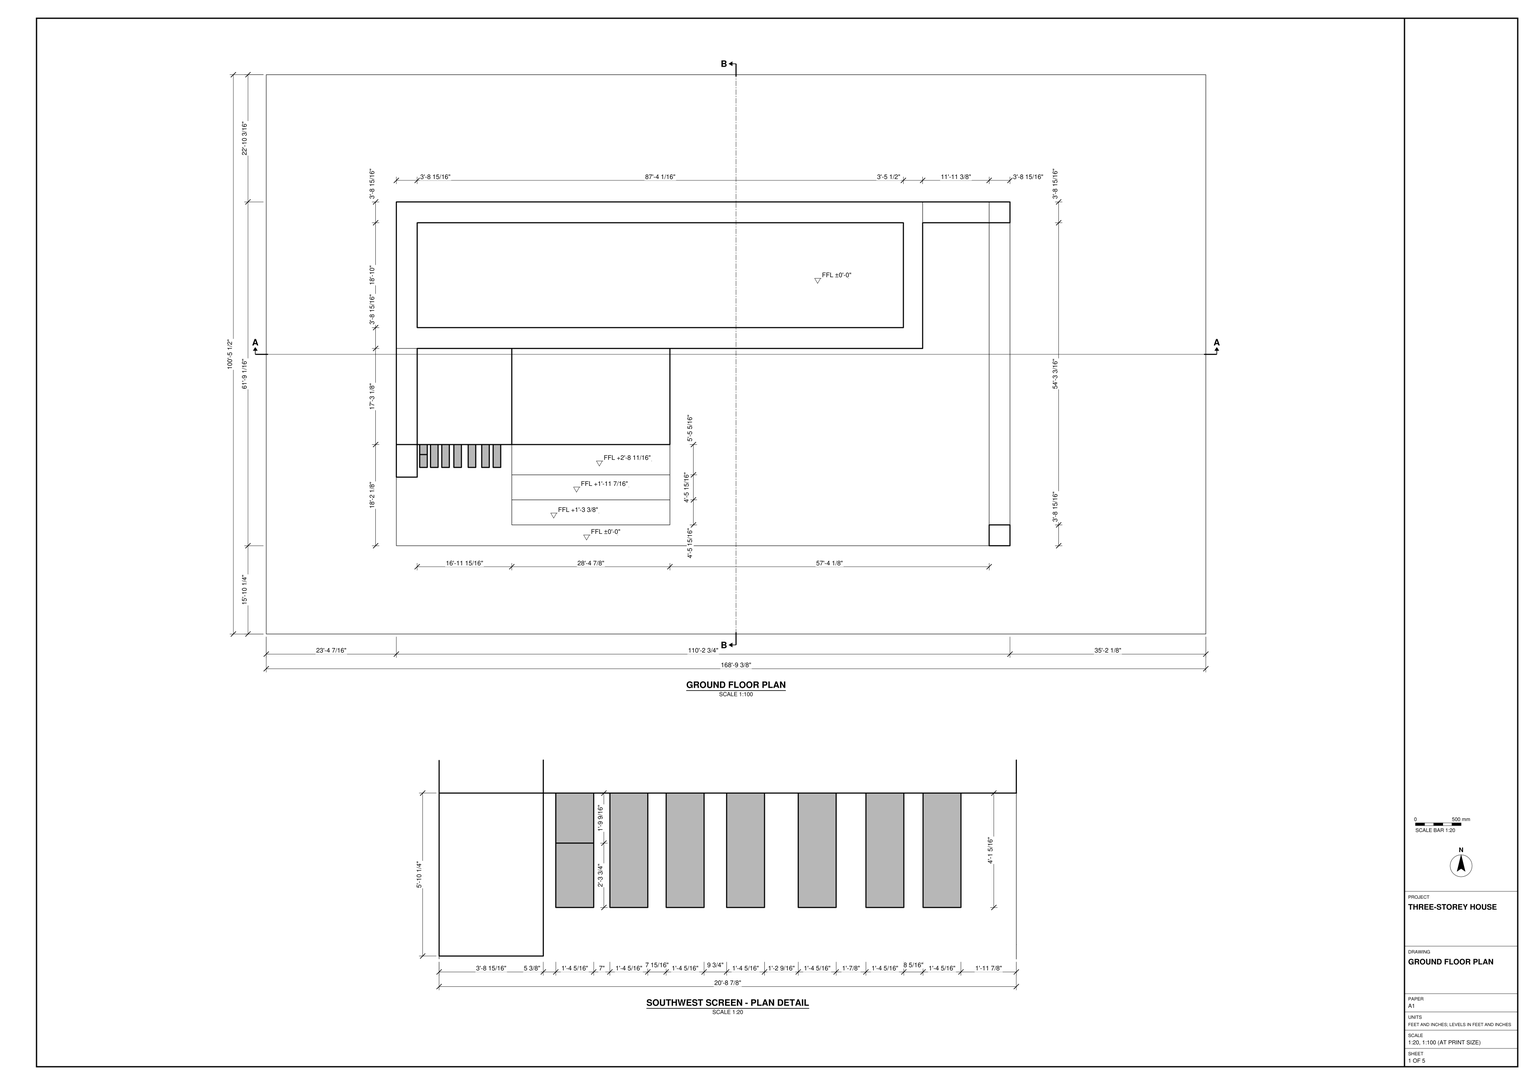
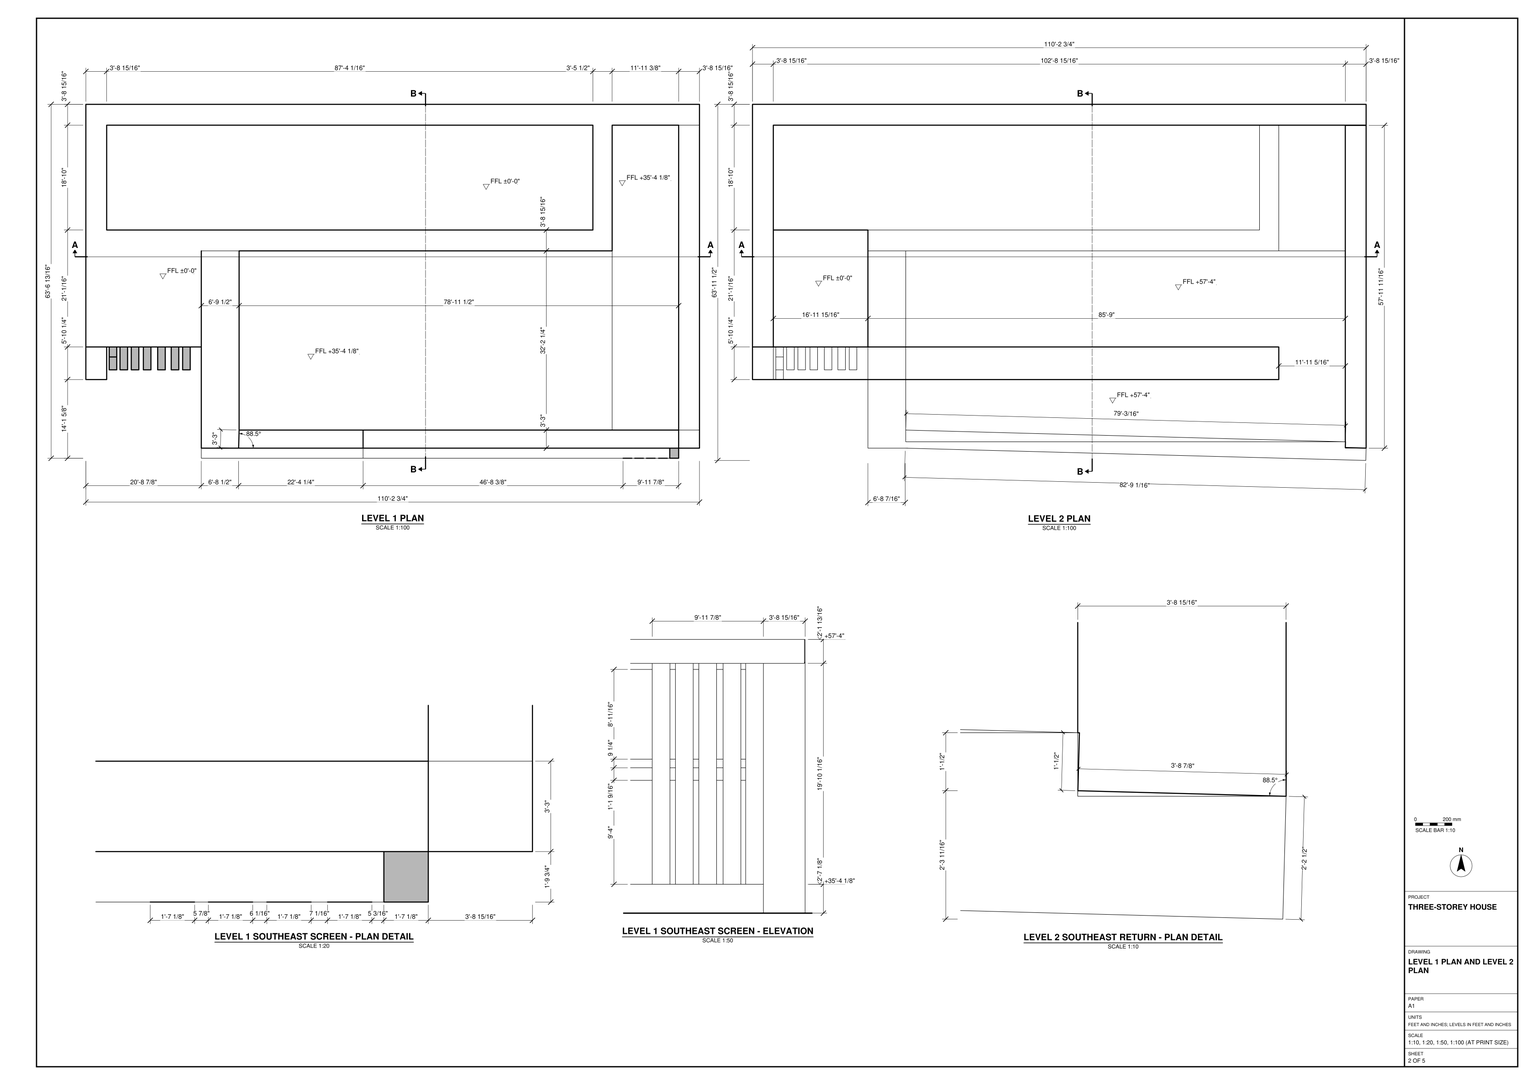
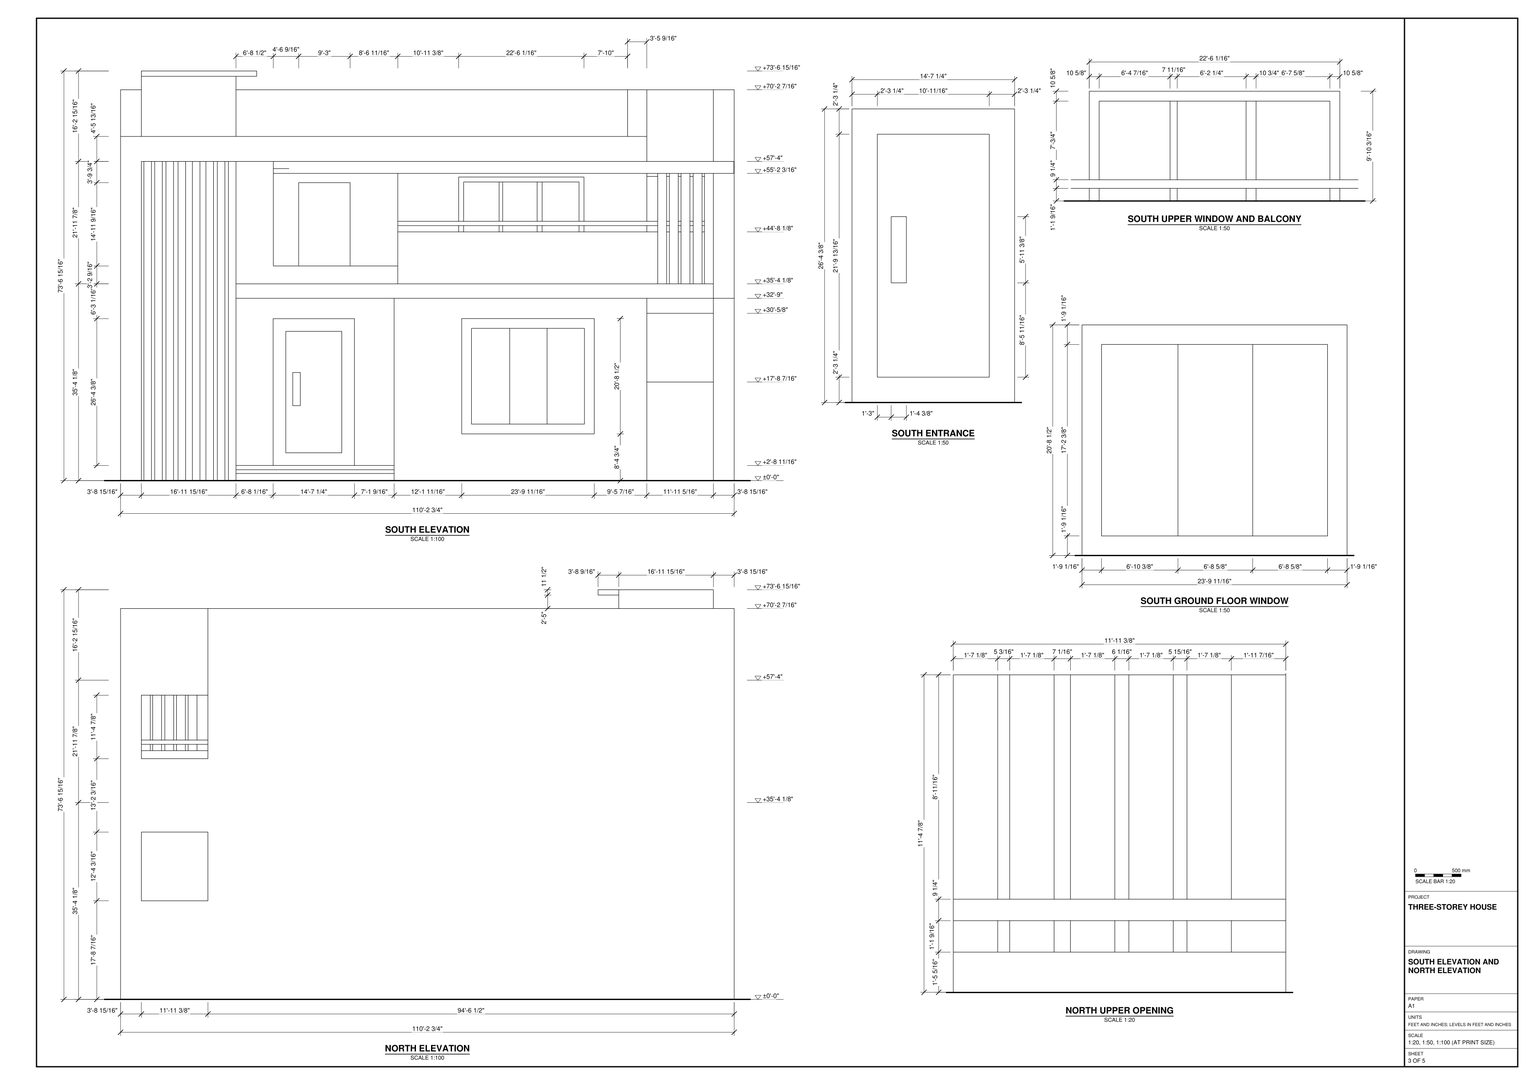
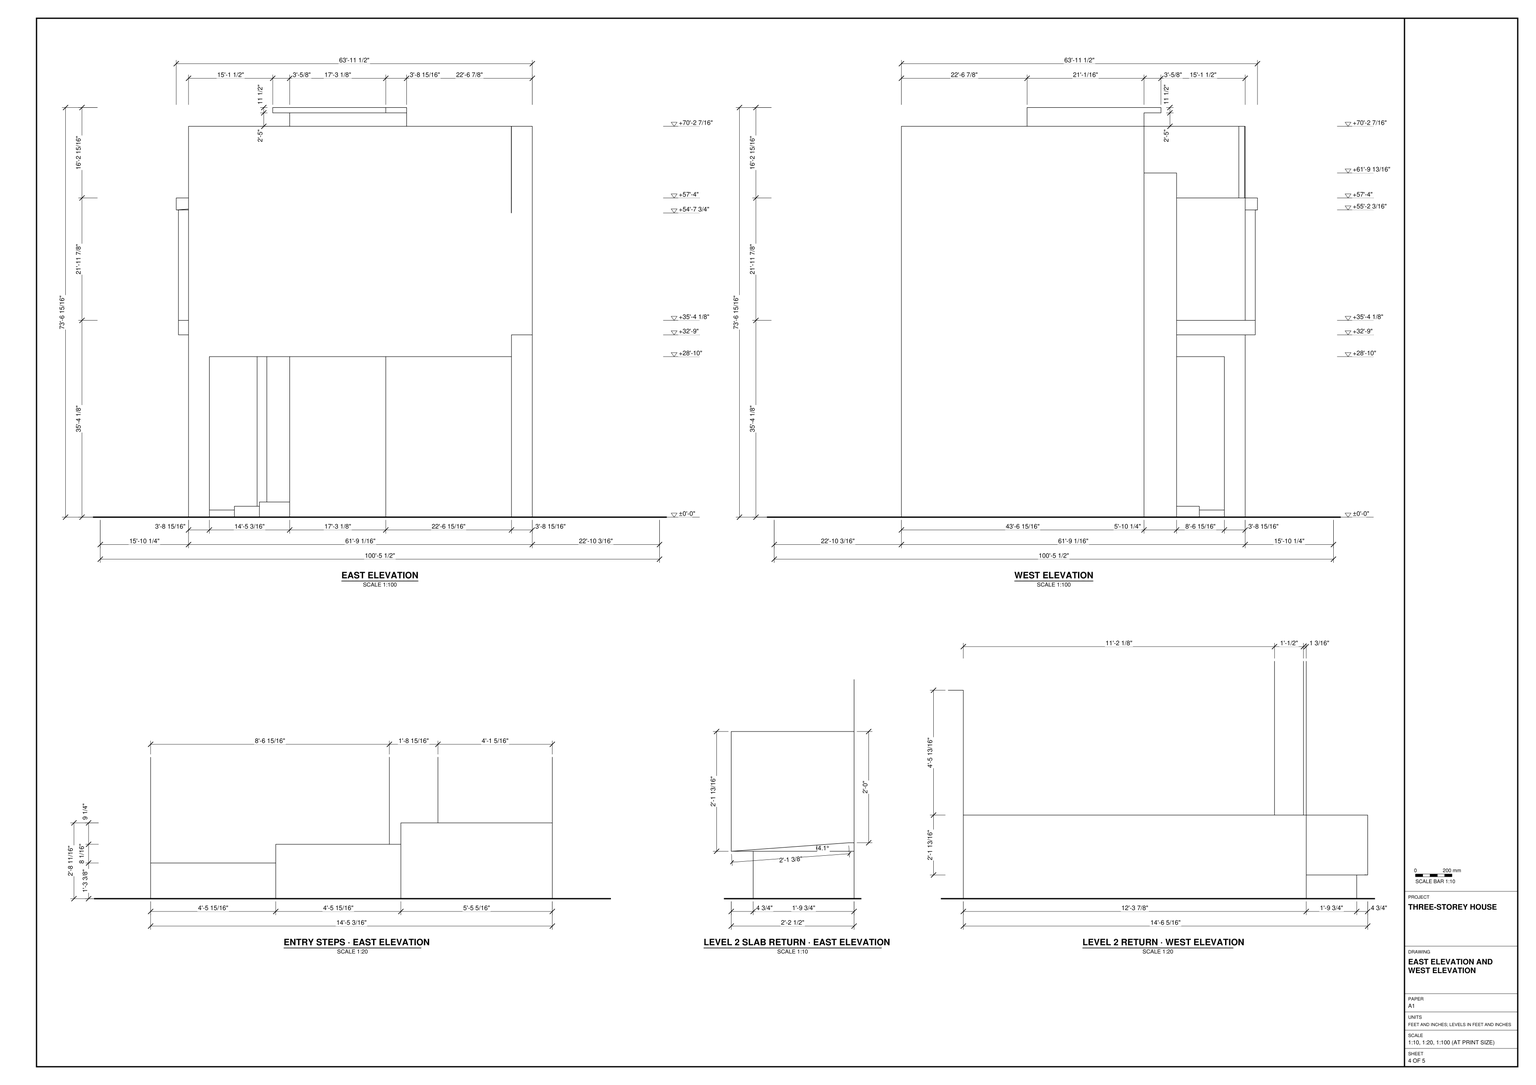
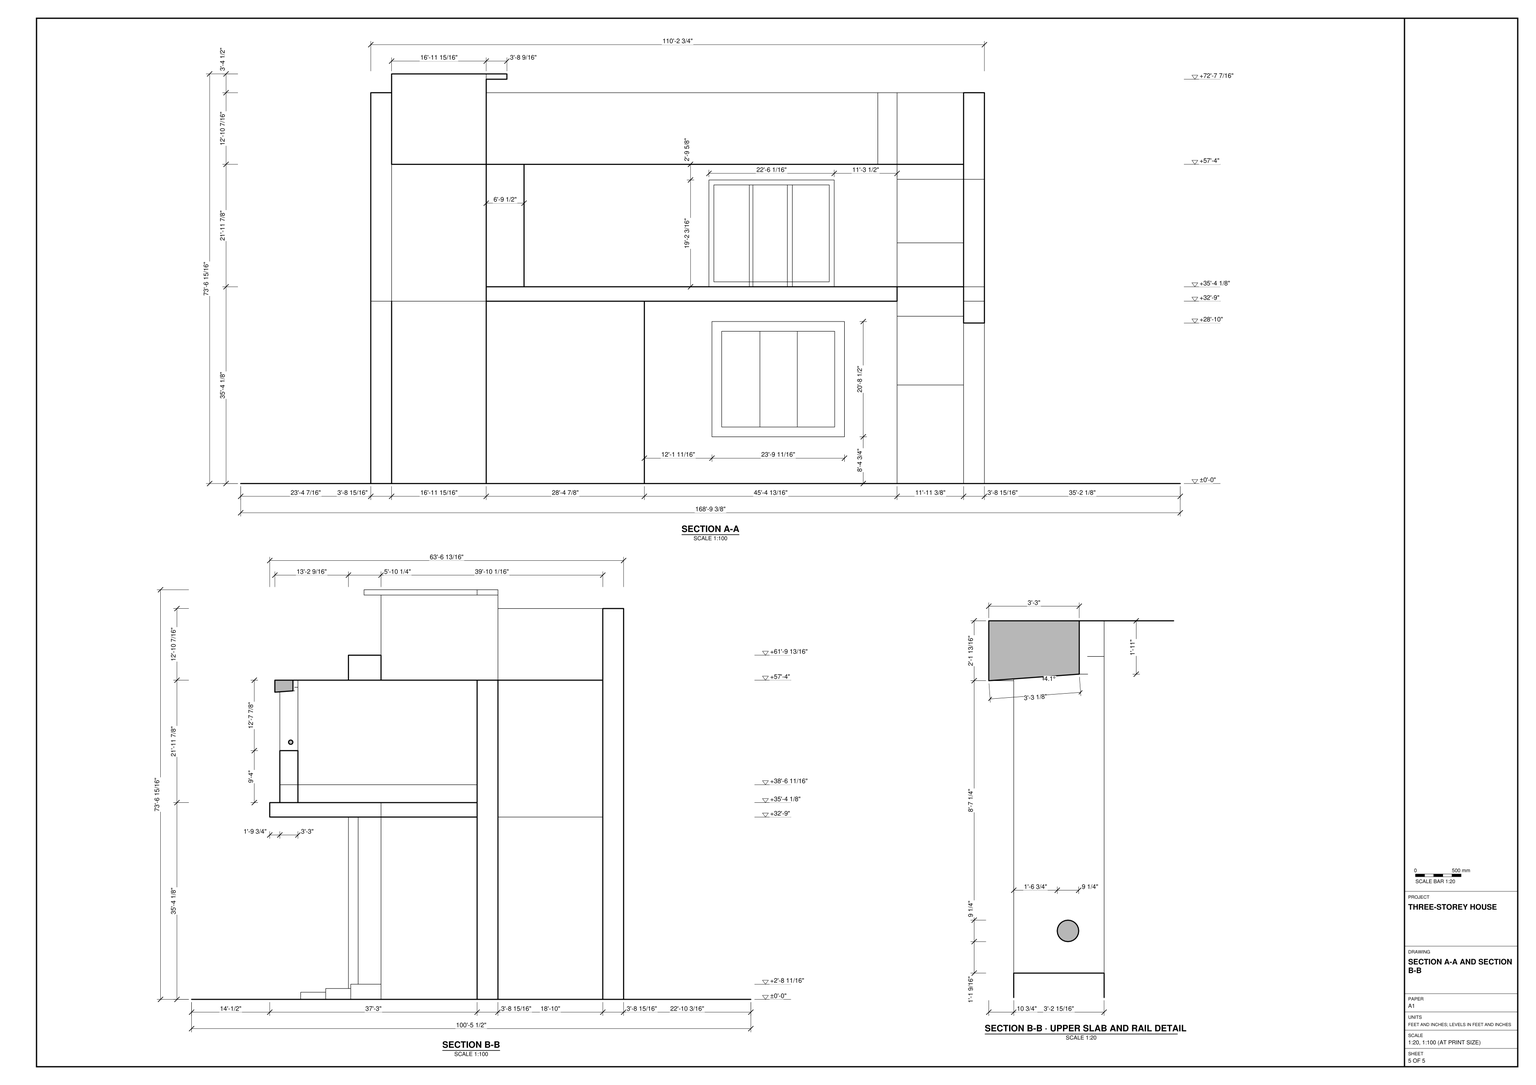
Build the three-storey house and its rectangular site base in SketchUp from task_files/diagram_01.pdf. Work in feet and inches. The overall model extents, including the base, are 168'-9 3/8" along X, 100'-5 1/2" along Y and 73'-6 15/16" along Z. Set the ground floor at ±0'-0", Level 1 at +35'-4 1/8" and Level 2 at +57'-4".

Position the house using the setbacks on the ground floor plan. Model the long rectangular space on the north side and follow the separate slab outlines and wall returns on the upper plans. Give the walls, floor slabs and roof their drawn thicknesses. Include the raised roof element and its projecting cap.

On the south side, run the broad entrance steps up to the framed door. Place the tall, spaced screen fins to the west of the steps and the divided ground floor window to the east of the door. Use the elevation details for the upper window, balcony edge and shorter southeast screen. On the north wall, align the lower opening with the screened opening above it. Include built-in joinery and main furniture only where shown. Decor and loose items may be any suitable library components.

Keep walls, slabs and roof elements in separate groups or components, group each furniture or joinery piece separately, and use components for repeated parts such as screen fins. Save one SketchUp model as output_files/three_storey_house_with_steps_and_vertical_screens.skp.

# SketchUp Ruby script. Lengths in inches.
U = 1.inch
M = Sketchup.active_model
def pt(a) = Geom::Point3d.new(a.map { |v| v * U })
def face(e, loops, mat)
  f = e.add_face(loops[0].map { |a| pt(a) })
  loops[1..].each { |l| e.add_face(l.map { |a| pt(a) }).erase! }
  f.material = f.back_material = mat if mat
  f
end
# faces: each face lists its corners as indices into pts; further lists are holes
def faces(e, pts, list, mat = nil) = list.each { |f| face(e, (f[0].is_a?(Array) ? f : [f]).map { |l| l.map { |i| pts[i] } }, mat) }
# xy, xz, yz: faces in a plane at the given z, y or x. An outline is a flat list of corners, or four numbers for a rectangle; further outlines are holes
def ring(l) = l.size == 4 ? [[l[0], l[1]], [l[2], l[1]], [l[2], l[3]], [l[0], l[3]]] : l.each_slice(2).to_a
def flat(e, list, mat, &to3) = list.each { |f| face(e, (f[0].is_a?(Array) ? f : [f]).map { |l| ring(l).map { |u, v| to3.(u, v) } }, mat) }
def xy(e, z, list, mat = nil) = flat(e, list, mat) { |x, y| [x, y, z] }
def xz(e, y, list, mat = nil) = flat(e, list, mat) { |x, z| [x, y, z] }
def yz(e, x, list, mat = nil) = flat(e, list, mat) { |y, z| [x, y, z] }
def lines(e, pts, list) = list.each { |a, b| e.add_line(pt(pts[a]), pt(pts[b])) }
# prism: a flat outline (further loops are holes) pulled along v
def prism(e, loops, v, mat = nil)
  f = face(e, loops, mat); d = Geom::Vector3d.new(v.map { |x| x * U })
  f.pushpull(f.normal.samedirection?(d) ? d.length : -d.length)
end
def box(e, o, s, mat = nil) = prism(e, [[o, [o[0] + s[0], o[1], o[2]], [o[0] + s[0], o[1] + s[1], o[2]], [o[0], o[1] + s[1], o[2]]]], [0, 0, s[2]], mat)
def at(x, y, z, deg = 0) = Geom::Transformation.translation(pt([x, y, z])) * Geom::Transformation.rotation(ORIGIN, Z_AXIS, deg.degrees)
def axes(o, x, y, z) = Geom::Transformation.new([*x, 0, *y, 0, *z, 0, *pt(o).to_a, 1])
def part(name) = M.definitions.add(name)
# library, detail: a bought-in or finely detailed component or shape, given as its bounding box
def library(name, o, s) = part(name).tap { |d| box(d.entities, o, s) }
def detail(e, o, s) = box(e.add_group.entities, o, s)
def put(e, d, t, mat = nil) = e.add_instance(d, t).tap { |i| i.material = mat if mat }
def group(e, t, mat = nil) = e.add_group.tap { |g| g.transformation = t; g.material = mat if mat }.entities
root = M.entities
M.materials.add("[0012_Bisque]").color = [255, 228, 196]
M.materials.add("[0013_LightCoral]").color = [240, 128, 128]
M.materials.add("[0014_DarkSalmon]").color = [233, 150, 122]
M.materials.add("[Blinds Weave]").color = [141, 91, 25]
M.materials.add("[Color M07]").color = [58, 58, 58]
M.materials.add("[Formica Beige]").color = [211, 187, 149]
M.materials.add("[Formica Graystone]").color = [149, 146, 135]
M.materials.add("[Mirror 01]").color = [185, 185, 185]
M.materials.add("[Quartz Light Brown]").color = [199, 184, 152]
M.materials.add("[Quartz Light Grey]").color = [251, 251, 252]
M.materials.add("[Translucent Glass Blue]").color = [100, 149, 237]
M.materials["[Translucent Glass Blue]"].alpha = 0.5
M.materials.add("[Translucent Glass Safety]").color = [204, 235, 244]
M.materials["[Translucent Glass Safety]"].alpha = 0.5
M.materials.add("[Window Covering 01]").color = [169, 163, 146]
M.materials.add("[Wood Bamboo]").color = [177, 105, 43]
M.materials.add("[Wood Floor Light]").color = [204, 176, 127]
M.materials.add("[Wood Lumber ButtJoined]").color = [164, 152, 112]
M.materials.add("[Wood OSB]").color = [240, 195, 122]
M.materials.add("[Wood Veneer 01]").color = [120, 70, 37]
xy(root,0,[[[0,0,2025.375,1205.5],[280.46,190.26,280.46,931.3,1558.31,931.3,1558.31,886.39,1603.22,886.39,1603.22,190.26]],[280.46,190.26,1558.31,190.26,1558.31,886.39,1414.96,886.39,1414.96,615.48,870.17,615.48,870.17,235.17,529.3125,235.17,529.3125,408.36,505.4375,408.36,505.4375,359.04,489.09,359.04,489.09,408.36,480.8125,408.36,480.8125,359.04,464.47,359.04,464.47,408.36,451.625,408.36,451.625,359.04,435.28,359.04,435.28,408.36,420.75,408.36,420.75,359.04,404.41,359.04,404.41,408.36,394.6875,408.36,394.6875,359.04,378.34,359.04,378.34,408.36,370.4375,408.36,370.4375,359.04,354.09,359.04,354.09,408.36,347.1,408.36,347.1,359.04,330.76,359.04,330.76,408.36,325.375,408.36,325.375,338.11,280.46,338.11],[1558.31,190.26,1603.22,235.17],[529.3125,235.17,870.17,289.12],[1558.31,235.17,1603.22,886.39],
  [529.3125,289.12,870.17,343.0625],[280.46,338.11,325.375,408.36],[529.3125,343.0625,870.17,408.36],[330.76,359.04,347.1,386.79],[354.09,359.04,370.4375,408.36],
  [378.34,359.04,394.6875,408.36],[404.41,359.04,420.75,408.36],[435.28,359.04,451.625,408.36],[464.47,359.04,480.8125,408.36],[489.09,359.04,505.4375,408.36],
  [330.76,386.79,347.1,408.36],[280.46,408.36,325.375,615.48],[325.375,408.36,529.3125,615.48],[529.3125,408.36,870.17,615.48],[[280.46,615.48,1414.96,931.3],[325.375,660.42,1373.43,886.39]],
  [325.375,660.42,1373.43,886.39],[1414.96,886.39,1558.31,931.3]])
xy(root,15.375,[[529.3125,235.17,870.17,289.12]],"[Quartz Light Brown]")
xy(root,23.4375,[[529.3125,289.12,870.17,343.0625]],"[Quartz Light Brown]")
xy(root,32.68,[[529.3125,343.0625,870.17,408.36]],"[Quartz Light Brown]")
xy(root,212.4375,[[1414.96,886.39,1558.31,931.3]])
xy(root,346.02,[[1558.31,235.17,1603.22,886.39]])
xy(root,360.625,[[1414.96,886.39,1558.31,931.3]])
xy(root,393,[[529.3125,168.51,870.17,408.36],[870.17,168.51,870.17,615.48,1414.96,615.48,1414.96,229.24,1558.31,229.24,1558.31,168.51],[529.3125,408.36,870.17,615.48]])
xy(root,424.13,[[529.3125,190.26,529.3125,615.48,610.83,615.48,610.83,229.24,1558.31,229.24,1558.31,190.26],[610.83,229.24,1414.96,615.48],[1414.96,229.24,1558.31,886.39]])
xy(root,424.13,[[529.3125,168.51,878.04,190.26],[878.04,168.51,1539.17,190.26],[1539.17,168.51,1558.31,190.26]],"[Quartz Light Grey]")
xy(root,462.69,[[609.79,190.26,610.83,229.24,878.04,229.24,878.04,190.26]])
xy(root,518.82,[[1414.96,886.39,1558.31,931.3]],"[0014_DarkSalmon]")
xy(root,536.13,[[878.04,190.26,1558.31,229.24]],"[Translucent Glass Blue]")
xy(root,655.67,[[1414.96,886.39,1558.31,931.3]],"[0014_DarkSalmon]")
xy(root,662.1875,[[1539.17,168.51,1558.31,190.26]],"[Quartz Light Grey]")
xy(root,664.02,[[1603.1875,189.0625,1558.31,190.26,1558.34,191.46,1603.22,190.26]])
xy(root,672.63,[[609.79,190.26,878.04,190.26,878.04,229.24,610.83,229.24]])
xy(root,688,[[1558.31,190.26,1558.34,191.46,1558.67,203.95,1558.31,203.96],[1558.31,190.26,1603.22,190.26,1558.34,191.46],[610.83,203.96,1558.31,203.96,610.83,229.24],[325.375,338.11,330.76,408.36],[330.76,338.11,347.1,359.04],
  [347.1,338.11,347.1,408.36,354.09,408.36,354.09,359.04,370.4375,359.04,370.4375,408.36,378.34,408.36,378.34,359.04,394.6875,359.04,394.6875,408.36,404.41,408.36,404.41,359.04,420.75,359.04,420.75,408.36,435.28,408.36,435.28,359.04,451.625,359.04,451.625,408.36,464.47,408.36,464.47,359.04,480.8125,359.04,480.8125,408.36,489.09,408.36,489.09,359.04,505.4375,359.04,505.4375,408.36,529.3125,408.36,529.3125,338.11],[529.3125,338.11,610.83,408.36],[330.76,359.04,347.1,386.79],[354.09,359.04,370.4375,408.36],[378.34,359.04,394.6875,408.36],
  [404.41,359.04,420.75,408.36],[435.28,359.04,451.625,408.36],[464.47,359.04,480.8125,408.36],[489.09,359.04,505.4375,408.36],[330.76,386.79,347.1,408.36],
  [325.375,408.36,529.3125,660.42],[529.3125,408.36,610.83,615.48],[529.3125,615.48,1414.96,615.48,1414.96,886.39,1373.43,886.39,1373.43,660.42,529.3125,660.42],[325.375,660.42,1373.43,886.39]])
xy(root,688,[[1414.96,615.48,1558.31,886.39]],"[0014_DarkSalmon]")
xy(root,688,[[1602.51,163.78,1603.22,190.26,1558.31,190.26,1558.31,203.96,610.83,203.96,610.83,338.11,529.3125,338.11,529.3125,190.26,609.79,190.26],[1558.31,203.96,1558.31,615.48,610.83,615.48,610.83,408.36,1415,408.36,1415,338.11,610.83,338.11,610.83,229.24]],"[Quartz Light Grey]")
xy(root,688,[[610.83,338.11,1415,408.36]],"[Wood Bamboo]")
xy(root,741.8125,[[280.46,338.11,1415,408.36]],"[0013_LightCoral]")
xy(root,842.4375,[[1603.22,190.26,1603.22,885.99,1558.31,885.99,1558.31,203.96,1558.67,203.95,1558.34,191.46],[280.46,408.36,325.375,408.36,325.375,886.39,1603.22,886.39,1603.22,931.3,280.46,931.3]],"[Formica Graystone]")
xy(root,871.46,[[325.375,371.73,573.875,408.36],[529.3125,408.36,573.875,615.48]])
xy(root,882.9375,[[325.375,371.73,573.875,371.73,573.875,615.48,529.3125,615.48,529.3125,660.42,325.375,660.42]],"[0012_Bisque]")
xz(root,168.51,[[529.3125,393,1558.31,424.13]],"[Quartz Light Grey]")
xz(root,168.51,[[1438.42,424.13,1457.56,662.1875],[1463.48,424.13,1482.62,662.1875],[1488.67,424.13,1507.81,662.1875],[1514.86,424.13,1534,662.1875],[1539.17,424.13,1558.31,662.1875]],"[Wood Floor Light]")
xz(root,190.26,[[1558.31,0,1603.22,393]],"[Formica Beige]")
xz(root,190.26,[[1558.31,393,1603.22,688],[529.3125,424.13,878.04,424.13,878.04,462.69,609.79,462.69,609.79,688,529.3125,688],[1539.17,536.13,1558.31,662.1875]],"[Quartz Light Grey]")
xz(root,190.26,[[878.04,424.13,1539.17,536.13],[1539.17,424.13,1558.31,536.13]],"[Translucent Glass Blue]")
xz(root,190.26,[[664.375,462.69,775.36,642.27]],"[Translucent Glass Safety]")
xz(root,190.26,[[609.79,462.69,664.375,462.69,664.375,642.27,775.36,642.27,775.36,462.69,878.04,462.69,878.04,672.63,609.79,672.63]],"[Wood Bamboo]")
xz(root,229.24,[[1414.96,393,1558.31,424.13]])
xz(root,229.24,[[610.83,424.13,610.83,462.69,878.04,462.69,878.04,536.13,1414.96,536.13,1414.96,424.13],[1414.96,424.13,1558.31,536.13]],"[Translucent Glass Blue]")
xz(root,229.24,[[610.83,462.69,878.04,672.63]],"[Wood Bamboo]")
xz(root,235.17,[[1558.31,0,1603.22,346.02]],"[Formica Beige]")
xz(root,235.17,[[529.3125,0,870.17,15.375]],"[Quartz Light Brown]")
xz(root,289.12,[[529.3125,0,870.17,15.375]])
xz(root,289.12,[[529.3125,15.375,870.17,23.4375]],"[Quartz Light Brown]")
xz(root,338.11,[[280.46,0,325.375,0,325.375,688,1415,688,1415,741.8125,280.46,741.8125]],"[0013_LightCoral]")
xz(root,343.0625,[[529.3125,0,870.17,23.4375]])
xz(root,343.0625,[[529.3125,23.4375,870.17,32.68]],"[Quartz Light Brown]")
xz(root,359.04,[[330.76,0,347.1,688],[354.09,0,370.4375,688],[378.34,0,394.6875,688],[404.41,0,420.75,688],[435.28,0,451.625,688],
  [464.47,0,480.8125,688],[489.09,0,505.4375,688]],"[Wood Lumber ButtJoined]")
xz(root,371.73,[[325.375,871.46,573.875,882.9375]],"[0012_Bisque]")
xz(root,386.79,[[330.76,0,347.1,688]])
xz(root,408.36,[[280.46,0,325.375,393],[325.375,0,330.76,688],[330.76,0,347.1,688],[354.09,0,370.4375,688],[378.34,0,394.6875,688],
  [404.41,0,420.75,688],[435.28,0,451.625,688],[464.47,0,480.8125,688],[489.09,0,505.4375,688],[529.3125,0,870.17,32.68],
  [280.46,393,325.375,741.8125],[325.375,688,529.3125,741.8125],[529.3125,688,1415,741.8125]])
xz(root,408.36,[[505.4375,0,512.97,688],[512.97,0,529.3125,688],[529.3125,32.68,609.35,32.68,609.35,349.05,784.6,349.05,784.6,32.68,870.17,32.68,870.17,393,529.3125,393],[325.375,741.8125,529.3125,871.46]],"[0012_Bisque]")
xz(root,408.36,[[280.46,741.8125,325.375,842.4375]],"[Formica Graystone]")
xz(root,408.36,[[[609.35,32.68,784.6,349.05],[636.625,59.95,757.33,321.78]],[[636.625,59.95,757.33,321.78],[651.61,161.62,667.99,233]]],"[Wood Bamboo]")
xz(root,408.36,[[347.1,0,354.09,688],[370.4375,0,378.34,688],[394.6875,0,404.41,688],[420.75,0,435.28,688],[451.625,0,464.47,688],
  [480.8125,0,489.09,688]],"[Wood Lumber ButtJoined]")
xz(root,408.36,[[651.61,161.62,667.99,233]],"[Wood OSB]")
xz(root,615.48,[[325.375,0,529.3125,393],[529.3125,0,870.17,393],[529.3125,393,1414.96,424.13]])
xz(root,615.48,[[[870.17,0,1414.96,393],[1015.85,100.76,1301.54,349.26]],[529.3125,871.46,573.875,882.9375]],"[0012_Bisque]")
xz(root,615.48,[[610.83,424.13,1009.38,424.13,1009.38,654.34,1279.43,654.34,1279.43,424.13,1414.96,424.13,1414.96,688,610.83,688]],"[0014_DarkSalmon]")
xz(root,615.48,[[1020.03,434.78,1096.49,643.69],[1104.17,434.78,1178.42,643.69],[1189.1875,434.78,1268.78,643.69]],"[Mirror 01]")
xz(root,615.48,[[1036.92,121.82,1119.27,328.19],[1119.27,121.82,1199.87,328.19],[1199.87,121.82,1280.47,328.19]],"[Window Covering 01]")
xz(root,615.48,[[1009.38,424.13,1096.49,424.13,1096.49,434.78,1020.03,434.78,1020.03,643.69,1268.78,643.69,1268.78,434.78,1189.1875,434.78,1189.1875,424.13,1279.43,424.13,1279.43,654.34,1009.38,654.34],[1096.49,424.13,1104.17,434.78],[1104.17,424.13,1178.42,434.78],[1178.42,424.13,1189.1875,434.78],[1096.49,434.78,1104.17,643.69],
  [1178.42,434.78,1189.1875,643.69]],"[Wood Bamboo]")
xz(root,615.48,[[[1015.85,100.76,1301.54,349.26],[1036.92,121.82,1280.47,328.19]]],"[Wood Veneer 01]")
xz(root,660.42,[[325.375,0,1373.43,393],[325.375,393,1373.43,688]])
xz(root,660.42,[[325.375,688,529.3125,882.9375]],"[0012_Bisque]")
xz(root,885.99,[[1558.31,655.73,1603.22,842.4375]])
xz(root,886.39,[[325.375,0,1373.43,393],[1558.31,346.02,1603.22,393],[1414.96,360.625,1558.31,424.13],[325.375,393,1373.43,688],[325.375,688,1373.43,842.4375],
  [1373.43,688,1414.96,842.4375],[1414.96,688,1558.31,842.4375]])
xz(root,886.39,[[1414.96,424.13,1558.31,518.82],[1414.96,655.67,1558.31,655.67,1558.31,655.73,1603.22,655.73,1603.22,842.4375,1558.31,842.4375,1558.31,688,1414.96,688]],"[Blinds Weave]")
xz(root,886.39,[[1414.96,0,1558.31,212.4375],[1558.31,0,1603.22,346.02]],"[Formica Beige]")
xz(root,931.3,[[[280.46,0,280.46,842.4375,1414.96,842.4375,1414.96,518.82,1558.31,518.82,1558.31,655.67,1414.96,655.67,1414.96,842.4375,1603.22,842.4375,1603.22,0],[1414.96,212.4375,1558.31,360.625]]],"[Formica Graystone]")
yz(root,280.46,[[338.11,0,408.36,741.8125]],"[0013_LightCoral]")
yz(root,280.46,[[408.36,0,931.3,842.4375]],"[Formica Graystone]")
yz(root,325.375,[[408.36,0,615.48,393],[660.42,0,886.39,393],[660.42,393,886.39,688],[408.36,688,660.42,842.4375],[660.42,688,886.39,842.4375]])
yz(root,325.375,[[408.36,842.4375,408.36,871.46,371.73,871.46,371.73,882.9375,660.42,882.9375,660.42,842.4375]],"[0012_Bisque]")
yz(root,325.375,[[338.11,0,408.36,688]],"[0013_LightCoral]")
yz(root,330.76,[[359.04,0,386.79,688],[386.79,0,408.36,688]])
yz(root,347.1,[[386.79,0,408.36,688]])
yz(root,347.1,[[359.04,0,386.79,688]],"[Wood Lumber ButtJoined]")
yz(root,354.09,[[359.04,0,408.36,688]],"[Wood Lumber ButtJoined]")
yz(root,370.4375,[[359.04,0,408.36,32.68],[359.04,32.68,408.36,393],[359.04,393,408.36,424.13],[359.04,424.13,408.36,688]],"[Wood Lumber ButtJoined]")
yz(root,378.34,[[359.04,0,408.36,688]],"[Wood Lumber ButtJoined]")
yz(root,394.6875,[[359.04,0,408.36,32.68],[359.04,32.68,408.36,393],[359.04,393,408.36,424.13],[359.04,424.13,408.36,688]],"[Wood Lumber ButtJoined]")
yz(root,404.41,[[359.04,0,408.36,688]],"[Wood Lumber ButtJoined]")
yz(root,420.75,[[359.04,0,408.36,32.68],[359.04,32.68,408.36,393],[359.04,393,408.36,424.13],[359.04,424.13,408.36,688]],"[Wood Lumber ButtJoined]")
yz(root,435.28,[[359.04,0,408.36,688]],"[Wood Lumber ButtJoined]")
yz(root,451.625,[[359.04,0,408.36,32.68],[359.04,32.68,408.36,393],[359.04,393,408.36,424.13],[359.04,424.13,408.36,688]],"[Wood Lumber ButtJoined]")
yz(root,464.47,[[359.04,0,408.36,688]],"[Wood Lumber ButtJoined]")
yz(root,480.8125,[[359.04,0,408.36,32.68],[359.04,32.68,408.36,393],[359.04,393,408.36,424.13],[359.04,424.13,408.36,688]],"[Wood Lumber ButtJoined]")
yz(root,489.09,[[359.04,0,408.36,688]],"[Wood Lumber ButtJoined]")
yz(root,505.4375,[[359.04,393,408.36,424.13],[359.04,424.13,408.36,688]])
yz(root,505.4375,[[359.04,0,408.36,32.68],[359.04,32.68,408.36,393]],"[Wood Lumber ButtJoined]")
yz(root,529.3125,[[408.36,0,615.48,393],[168.51,393,408.36,424.13],[408.36,393,615.48,424.13],[190.26,424.13,408.36,688],[408.36,424.13,615.48,688]])
yz(root,529.3125,[[408.36,688,660.42,871.46],[615.48,871.46,660.42,882.9375]],"[0012_Bisque]")
yz(root,529.3125,[[235.17,0,289.12,15.375],[289.12,0,343.0625,23.4375],[343.0625,0,408.36,32.68]],"[Quartz Light Brown]")
yz(root,573.875,[[371.73,871.46,615.48,882.9375]],"[0012_Bisque]")
yz(root,610.83,[[229.24,424.13,615.48,462.69],[229.24,462.69,615.48,688]],"[0014_DarkSalmon]")
yz(root,870.17,[[408.36,0,615.48,393]],"[0012_Bisque]")
yz(root,870.17,[[235.17,0,289.12,15.375],[289.12,0,343.0625,23.4375],[343.0625,0,408.36,32.68]],"[Quartz Light Brown]")
yz(root,878.04,[[190.26,462.69,229.24,536.13]])
yz(root,878.04,[[[190.26,536.13,229.24,672.63],[213.65,549.7,212.45,549.86,211.34,550.32,210.38,551.06,209.64,552.02,209.18,553.13,209.03,554.33,209.18,555.52,209.64,556.64,210.38,557.6,211.34,558.33,212.45,558.8,213.65,558.95,214.85,558.8,215.96,558.33,216.92,557.6,217.66,556.64,218.12,555.52,218.28,554.33,218.12,553.13,217.66,552.02,216.92,551.06,215.96,550.32,214.85,549.86]]],"[Wood Bamboo]")
yz(root,1373.43,[[660.42,0,886.39,393],[660.42,393,886.39,688]])
yz(root,1414.96,[[886.39,212.4375,931.3,360.625],[229.24,393,615.48,424.13],[615.48,393,660.42,424.13],[660.42,393,886.39,424.13]])
yz(root,1414.96,[[615.48,0,886.39,393]],"[0012_Bisque]")
yz(root,1414.96,[[615.48,424.13,660.42,688],[660.42,424.13,886.39,688],[886.39,518.82,931.3,655.67]],"[0014_DarkSalmon]")
yz(root,1415,[[338.11,688,408.36,741.8125]])
yz(root,1539.17,[[168.51,424.13,190.26,662.1875]],"[Quartz Light Grey]")
yz(root,1558.31,[[886.39,212.4375,931.3,360.625],[190.26,424.13,229.24,536.13],[213.65,549.7,214.85,549.86,215.96,550.32,216.92,551.06,217.66,552.02,218.12,553.13,218.28,554.33,218.12,555.52,217.66,556.64,216.92,557.6,215.96,558.33,214.85,558.8,213.65,558.95,212.45,558.8,211.34,558.33,210.38,557.6,209.64,556.64,209.18,555.52,209.03,554.33,209.18,553.13,209.64,552.02,210.38,551.06,211.34,550.32,212.45,549.86],[203.96,688,615.48,842.4375],[615.48,688,885.99,842.4375]])
yz(root,1558.31,[[886.39,518.82,931.3,655.67]],"[0014_DarkSalmon]")
yz(root,1558.31,[[229.24,424.13,886.39,655.73],[[190.26,536.13,190.26,688,885.99,688,885.99,655.73,229.24,655.73,229.24,536.13],[213.65,549.7,214.85,549.86,215.96,550.32,216.92,551.06,217.66,552.02,218.12,553.13,218.28,554.33,218.12,555.52,217.66,556.64,216.92,557.6,215.96,558.33,214.85,558.8,213.65,558.95,212.45,558.8,211.34,558.33,210.38,557.6,209.64,556.64,209.18,555.52,209.03,554.33,209.18,553.13,209.64,552.02,210.38,551.06,211.34,550.32,212.45,549.86]]],"[Blinds Weave]")
yz(root,1558.31,[[190.26,0,190.26,393,229.24,393,229.24,424.13,886.39,424.13,886.39,346.02,235.17,346.02,235.17,0]],"[Formica Beige]")
yz(root,1558.31,[[168.51,393,190.26,424.13],[168.51,424.13,190.26,662.1875]],"[Quartz Light Grey]")
yz(root,1603.22,[[886.39,0,931.3,393]],"[Formica Beige]")
yz(root,1603.22,[[190.26,0,235.17,0,235.17,346.02,886.39,346.02,886.39,393,931.3,393,931.3,842.4375,886.39,842.4375,886.39,655.73,885.99,655.73,885.99,842.4375,190.26,842.4375]],"[Formica Graystone]")
p = [[610.83,229.24,665.01],[610.83,229.24,462.69],[609.79,190.26,462.69],[609.79,190.26,662.1875],[1558.31,213.65,549.7],[1558.31,212.45,549.86],
  [878.04,212.45,549.86],[878.04,213.65,549.7],[1558.31,214.85,549.86],[878.04,214.85,549.86],[1558.31,211.34,550.32],[878.04,211.34,550.32],
  [1558.31,215.96,550.32],[878.04,215.96,550.32],[1558.31,210.38,551.06],[878.04,210.38,551.06],[1558.31,216.92,551.06],[878.04,216.92,551.06],
  [1558.31,209.64,552.02],[878.04,209.64,552.02],[1558.31,217.66,552.02],[878.04,217.66,552.02],[1558.31,209.18,553.13],[878.04,209.18,553.13],
  [1558.31,218.12,553.13],[878.04,218.12,553.13],[1558.31,209.03,554.33],[878.04,209.03,554.33],[1558.31,218.28,554.33],[878.04,218.28,554.33],
  [1558.31,209.18,555.52],[878.04,209.18,555.52],[1558.31,218.12,555.52],[878.04,218.12,555.52],[1558.31,209.64,556.64],[878.04,209.64,556.64],
  [1558.31,217.66,556.64],[878.04,217.66,556.64],[1558.31,210.38,557.6],[878.04,210.38,557.6],[1558.31,216.92,557.6],[878.04,216.92,557.6],
  [1558.31,211.34,558.33],[878.04,211.34,558.33],[1558.31,215.96,558.33],[878.04,215.96,558.33],[1558.31,212.45,558.8],[878.04,212.45,558.8],
  [1558.31,214.85,558.8],[878.04,214.85,558.8],[1558.31,213.65,558.95],[878.04,213.65,558.95],[609.79,190.26,672.63],[1602.51,163.78,662.1875],
  [1602.51,163.78,688],[609.79,190.26,688],[1558.31,203.96,665.01],[1558.67,203.95,665.01],[1558.34,191.46,664.1],[1558.31,190.26,664.02],
  [1603.1875,189.0625,664.02],[1603.22,190.26,664.02],[1603.22,190.26,688],[610.83,229.24,672.63],[1558.34,191.46,688],[1558.31,190.26,688],
  [1558.34,191.46,664.02],[1558.67,203.95,688],[610.83,229.24,688],[1558.31,203.96,688],[1603.22,190.26,842.4375],[1558.34,191.46,842.4375],
  [1558.67,203.95,842.4375],[1558.31,203.96,842.4375],[280.46,615.48,393],[325.375,615.48,393],[1414.96,886.39,393],[1414.96,931.3,393],
  [1558.31,886.39,393],[1558.31,931.3,393],[1558.31,229.24,424.13],[1603.22,229.24,424.13],[1558.31,886.39,424.13],[1603.22,886.39,424.13],
  [1558.31,229.24,655.73],[1603.22,229.24,655.73]]
faces(root,p,[[0,1,2,3],[3,0,56,57,58,59,60,53],[53,60,61,62,54],[63,0,3,52],[59,58,64,65],[66,58,64,62,61],[66,59,58],[67,64,58,57],
  [68,69,56,0,63],[57,56,69,67],[67,64,71,72],[69,67,72,73]])
faces(root,p,[[4,5,6,7],[8,4,7,9],[5,10,11,6],[12,8,9,13],[10,14,15,11],[16,12,13,17],[14,18,19,15],[20,16,17,21],
  [18,22,23,19],[24,20,21,25],[22,26,27,23],[28,24,25,29],[26,30,31,27],[32,28,29,33],[30,34,35,31],[36,32,33,37],
  [34,38,39,35],[40,36,37,41],[38,42,43,39],[44,40,41,45],[42,46,47,43],[48,44,45,49],[46,50,51,47],[50,48,49,51]],"[Color M07]")
faces(root,p,[[52,3,53,54,55]],"[Quartz Light Grey]")
faces(root,p,[[64,62,70,71]],"[Formica Graystone]")
lines(root,p,[[74,75],[76,77],[78,79],[80,81],[82,83],[84,85]])
